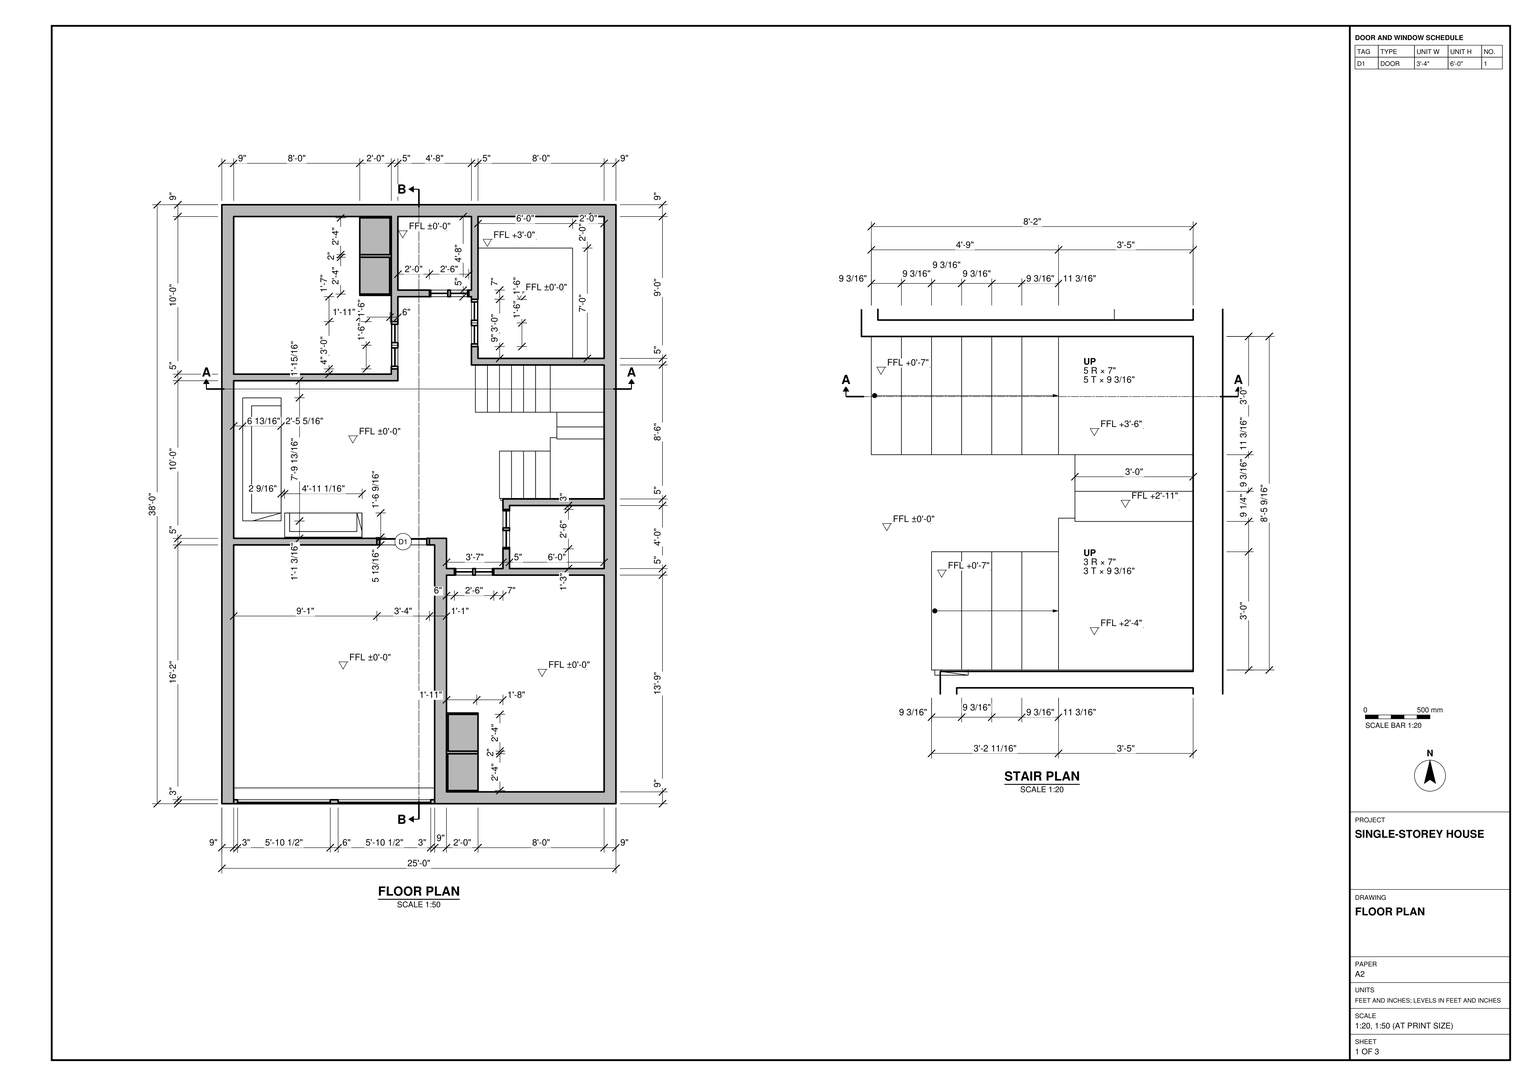
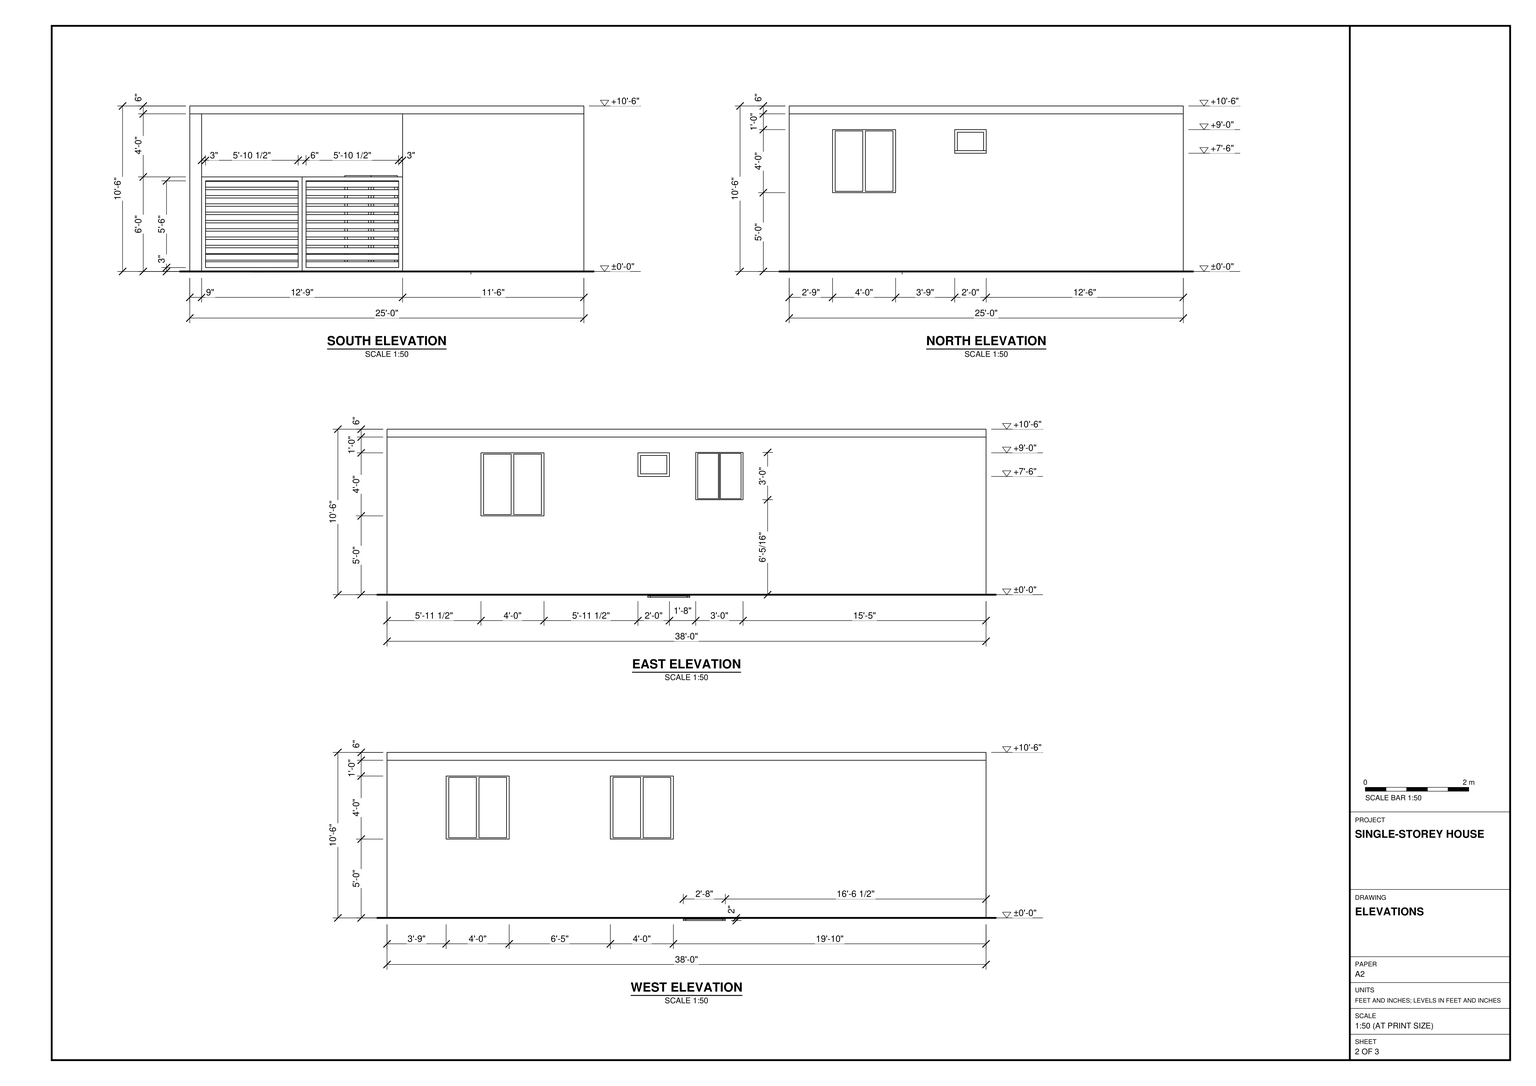
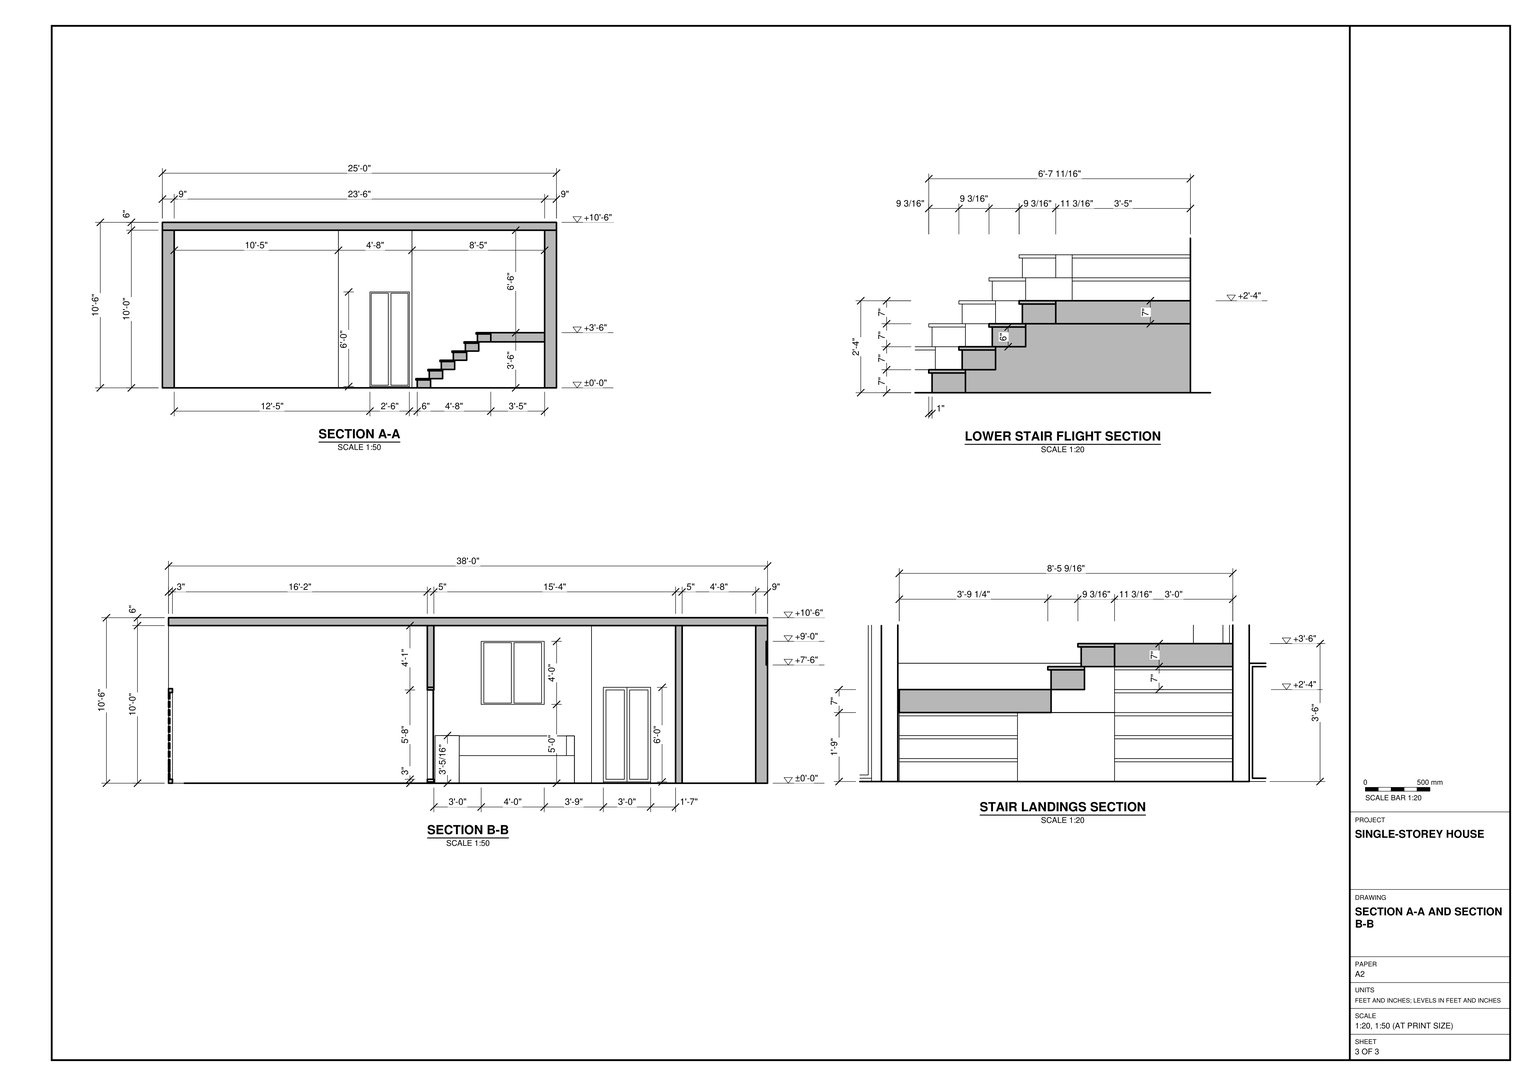
Build the single-storey house in SketchUp using task_files/diagram_01.pdf. Work in feet and inches. Set the ground-floor level at ±0'-0". The house measures 25'-0" east to west and 38'-0" north to south, with an overall model height of 10'-8".

Use the floor plan to lay out the two large southern rooms, the central space, the northern rooms and the small room immediately south of the stairs. Model the floor slab, walls at their drawn thicknesses, and flat roof slab. Fit the scheduled door in the partition between the southwest room and the central space. Use the elevations to position the windows and the paired slatted panels on the south face.

Build the two stair flights on the east side of the central space. Follow the enlarged plan and sections for the treads, risers and steps connecting the landings. Include the raised area in the northeast room, the low units arranged at right angles in the central space and the paired rectangular units in the northwest and southeast rooms.

Keep shell elements such as walls, slabs and roof, and each furniture or joinery piece, in separate groups or components. Use components for repeated parts. Decor and loose items may be represented by any suitable library component. Save one SketchUp model as output_files/single_storey_house_with_paired_stair_flights.skp.

# SketchUp Ruby script. Lengths in inches.
U = 1.inch
M = Sketchup.active_model
def pt(a) = Geom::Point3d.new(a.map { |v| v * U })
def face(e, loops, mat)
  f = e.add_face(loops[0].map { |a| pt(a) })
  loops[1..].each { |l| e.add_face(l.map { |a| pt(a) }).erase! }
  f.material = f.back_material = mat if mat
  f
end
# faces: each face lists its corners as indices into pts; further lists are holes
def faces(e, pts, list, mat = nil) = list.each { |f| face(e, (f[0].is_a?(Array) ? f : [f]).map { |l| l.map { |i| pts[i] } }, mat) }
# xy, xz, yz: faces in a plane at the given z, y or x. An outline is a flat list of corners, or four numbers for a rectangle; further outlines are holes
def ring(l) = l.size == 4 ? [[l[0], l[1]], [l[2], l[1]], [l[2], l[3]], [l[0], l[3]]] : l.each_slice(2).to_a
def flat(e, list, mat, &to3) = list.each { |f| face(e, (f[0].is_a?(Array) ? f : [f]).map { |l| ring(l).map { |u, v| to3.(u, v) } }, mat) }
def xy(e, z, list, mat = nil) = flat(e, list, mat) { |x, y| [x, y, z] }
def xz(e, y, list, mat = nil) = flat(e, list, mat) { |x, z| [x, y, z] }
def yz(e, x, list, mat = nil) = flat(e, list, mat) { |y, z| [x, y, z] }
def lines(e, pts, list) = list.each { |a, b| e.add_line(pt(pts[a]), pt(pts[b])) }
# prism: a flat outline (further loops are holes) pulled along v
def prism(e, loops, v, mat = nil)
  f = face(e, loops, mat); d = Geom::Vector3d.new(v.map { |x| x * U })
  f.pushpull(f.normal.samedirection?(d) ? d.length : -d.length)
end
def box(e, o, s, mat = nil) = prism(e, [[o, [o[0] + s[0], o[1], o[2]], [o[0] + s[0], o[1] + s[1], o[2]], [o[0], o[1] + s[1], o[2]]]], [0, 0, s[2]], mat)
def at(x, y, z, deg = 0) = Geom::Transformation.translation(pt([x, y, z])) * Geom::Transformation.rotation(ORIGIN, Z_AXIS, deg.degrees)
def axes(o, x, y, z) = Geom::Transformation.new([*x, 0, *y, 0, *z, 0, *pt(o).to_a, 1])
def part(name) = M.definitions.add(name)
# library, detail: a bought-in or finely detailed component or shape, given as its bounding box
def library(name, o, s) = part(name).tap { |d| box(d.entities, o, s) }
def detail(e, o, s) = box(e.add_group.entities, o, s)
def put(e, d, t, mat = nil) = e.add_instance(d, t).tap { |i| i.material = mat if mat }
def group(e, t, mat = nil) = e.add_group.tap { |g| g.transformation = t; g.material = mat if mat }.entities
root = M.entities
M.materials.add("[Blinds Vertical Pattern]").color = [212, 212, 214]
M.materials.add("[Blinds Vertical Stripe Gray]").color = [160, 160, 160]
M.materials.add("[Blinds Wood Light]").color = [155, 100, 14]
M.materials.add("[Field Square Tile]").color = [217, 201, 169]
M.materials.add("[Granite Tile]").color = [155, 148, 143]
M.materials.add("[Marble Carrara Floor Tile]").color = [204, 208, 219]
M.materials.add("[Marble Carrara Gold Floor Tile]").color = [225, 223, 217]
M.materials.add("[Metal Aluminum Anodized]").color = [202, 209, 219]
M.materials.add("[Metal Rusted]").color = [184, 117, 91]
M.materials.add("[Translucent Glass Tinted]").color = [8, 201, 241]
M.materials["[Translucent Glass Tinted]"].alpha = 0.48
M.materials.add("[Wood Cherry Original]").color = [152, 86, 42]
M.materials.add("[Wood Floor Parquet]").color = [145, 89, 39]
M.materials.add("[Wood OSB]").color = [240, 195, 122]
c1 = part("Window sill \#1")
box(c1.entities,[0,0,0],[40,5,1])
c2 = part("Two-panel window")
xy(c2.entities,0,[[0,-2.5,30,2.5]],"[Blinds Wood Light]")
xy(c2.entities,1,[[1,-2.5,14,0],[16,-2.5,29,0],[1,0,14,2.5],[16,0,29,2.5]],"[Blinds Wood Light]")
xy(c2.entities,71,[[1,-2.5,14,0],[16,-2.5,29,0],[1,0,14,2.5],[16,0,29,2.5]],"[Blinds Wood Light]")
xy(c2.entities,72,[[0,-2.5,30,2.5]],"[Blinds Wood Light]")
xz(c2.entities,-2.5,[[[0,0,30,72],[16,1,29,71],[1,1,14,71]]],"[Blinds Wood Light]")
xz(c2.entities,0,[[1,1,14,71],[16,1,29,71]],"[Blinds Wood Light]")
xz(c2.entities,2.5,[[[0,0,30,72],[16,1,29,71],[1,1,14,71]]],"[Blinds Wood Light]")
yz(c2.entities,0,[[-2.5,0,2.5,72]],"[Blinds Wood Light]")
yz(c2.entities,1,[[-2.5,1,0,71],[0,1,2.5,71]],"[Blinds Wood Light]")
yz(c2.entities,14,[[-2.5,1,0,71],[0,1,2.5,71]],"[Blinds Wood Light]")
yz(c2.entities,16,[[-2.5,1,0,71],[0,1,2.5,71]],"[Blinds Wood Light]")
yz(c2.entities,29,[[-2.5,1,0,71],[0,1,2.5,71]],"[Blinds Wood Light]")
yz(c2.entities,30,[[-2.5,0,2.5,72]],"[Blinds Wood Light]")
c3 = part("Window sill")
xy(c3.entities,0,[[0,0,30,5]],"[Marble Carrara Gold Floor Tile]")
xy(c3.entities,1,[[0,0,30,5]],"[Wood OSB]")
xz(c3.entities,0,[[0,0,30,1]],"[Wood OSB]")
xz(c3.entities,5,[[0,0,30,1]],"[Wood OSB]")
yz(c3.entities,0,[[0,0,5,1]],"[Marble Carrara Gold Floor Tile]")
yz(c3.entities,30,[[0,0,5,1]],"[Marble Carrara Gold Floor Tile]")
c4 = part("Window sash")
xy(c4.entities,0,[[0,0,1,24]],"[Blinds Vertical Pattern]")
xy(c4.entities,2,[[0,2,1,22]],"[Blinds Vertical Pattern]")
xy(c4.entities,16,[[0,2,1,22]],"[Blinds Vertical Pattern]")
xy(c4.entities,18,[[0,0,1,24]],"[Blinds Vertical Pattern]")
xz(c4.entities,0,[[0,0,1,18]],"[Blinds Vertical Pattern]")
xz(c4.entities,2,[[0,2,1,16]],"[Blinds Vertical Pattern]")
xz(c4.entities,22,[[0,2,1,16]],"[Blinds Vertical Pattern]")
xz(c4.entities,24,[[0,0,1,18]],"[Blinds Vertical Pattern]")
yz(c4.entities,0,[[[0,0,24,18],[2,2,22,16]]],"[Blinds Vertical Pattern]")
yz(c4.entities,0,[[2,2,22,16]],"[Blinds Vertical Stripe Gray]")
yz(c4.entities,1,[[[0,0,24,18],[2,2,22,16]]],"[Blinds Vertical Pattern]")
c5 = part("Stair step")
xy(c5.entities,0,[[0,0,10.17,36]],"[Marble Carrara Gold Floor Tile]")
xy(c5.entities,6,[[0,0,10.17,36]],"[Granite Tile]")
xz(c5.entities,0,[[0,0,10.17,6]],"[Granite Tile]")
xz(c5.entities,36,[[0,0,10.17,6]],"[Marble Carrara Gold Floor Tile]")
yz(c5.entities,0,[[0,0,36,6]],"[Granite Tile]")
yz(c5.entities,10.17,[[0,0,36,6]],"[Granite Tile]")
c6 = part("Group\#4")
xy(c6.entities,0,[[0,-3.5,48,5.5]])
xy(c6.entities,1,[[2,-3.5,23,1],[25,-3.5,46,1],[2,1,23,5.5],[25,1,46,5.5]],"[Wood Cherry Original]")
xy(c6.entities,47,[[2,-3.5,23,1],[25,-3.5,46,1],[2,1,23,5.5],[25,1,46,5.5]],"[Wood Cherry Original]")
xy(c6.entities,48,[[0,-3.5,48,5.5]],"[Wood Cherry Original]")
xz(c6.entities,-3.5,[[[0,0,48,48],[2,1,23,47],[25,1,46,47]]],"[Wood Cherry Original]")
xz(c6.entities,1,[[2,1,23,47],[25,1,46,47]],"[Translucent Glass Tinted]")
xz(c6.entities,5.5,[[[0,0,48,48],[2,1,23,47],[25,1,46,47]]],"[Wood Cherry Original]")
yz(c6.entities,0,[[-3.5,0,5.5,48]],"[Wood Cherry Original]")
yz(c6.entities,2,[[-3.5,1,1,47],[1,1,5.5,47]],"[Wood Cherry Original]")
yz(c6.entities,23,[[-3.5,1,1,47],[1,1,5.5,47]],"[Wood Cherry Original]")
yz(c6.entities,25,[[-3.5,1,1,47],[1,1,5.5,47]],"[Wood Cherry Original]")
yz(c6.entities,46,[[-3.5,1,1,47],[1,1,5.5,47]],"[Wood Cherry Original]")
yz(c6.entities,48,[[-3.5,0,5.5,48]],"[Wood Cherry Original]")
c7 = part("Framing strip")
box(c7.entities,[0,-1,-2],[70.5,1,4.41])
c8 = part("Group\#1")
g1 = group(c8.entities,at(0,0,0))
xy(g1,0,[[0,0,5,36]],"[Marble Carrara Gold Floor Tile]")
xy(g1,1,[[0,0,5,36]],"[Wood OSB]")
xz(g1,0,[[0,0,5,1]],"[Marble Carrara Gold Floor Tile]")
xz(g1,36,[[0,0,5,1]],"[Marble Carrara Gold Floor Tile]")
yz(g1,0,[[0,0,36,1]],"[Wood OSB]")
yz(g1,5,[[0,0,36,1]],"[Wood OSB]")
c9 = part("Group\#9")
box(c9.entities,[-1,0,0],[11.17,36,1])
c10 = part("Rectangular panel")
box(c10.entities,[1,-28,0],[22,28,1])
c11 = part("Group\#14")
yz(c11.entities,0,[[0,0,28,70]])
c12 = part("Group\#13")
xy(c12.entities,0,[[-24,0,0,60]])
xy(c12.entities,1,[[-24,1,-1.25,29],[-24,31,-1,59]])
xy(c12.entities,71,[[-24,1,-1.25,29],[-24,31,-1,59]])
xy(c12.entities,72,[[-24,0,0,60]])
xz(c12.entities,0,[[-24,0,0,72]])
xz(c12.entities,1,[[-24,1,-1.25,71]])
xz(c12.entities,29,[[-24,1,-1.25,71]])
xz(c12.entities,31,[[-24,1,-1,71]])
xz(c12.entities,59,[[-24,1,-1,54.74],[-24,54.74,-1,55.74],[-24,55.74,-1,71]])
xz(c12.entities,60,[[-24,0,0,72]])
yz(c12.entities,-24,[[[0,0,60,72],[1,1,29,71],[31,1,59,71]]])
yz(c12.entities,-1.25,[[1,1,29,71]])
yz(c12.entities,-1,[[31,1,59,71]])
yz(c12.entities,0,[[0,0,60,72]])
p = [[-24,29.99,-0.01],[-24,29.99,0],[-24,60.01,72.01],[-24,60.01,-0.01],[-24,29.99,72],[-24,29.99,72.01]]
lines(c12.entities,p,[[0,1],[2,3],[3,0],[4,5]])
put(c12.entities,c10,at(-24,59,70))
put(c12.entities,c10,at(-24,59,56.2))
put(c12.entities,c10,at(-24,59,42.4))
put(c12.entities,c10,at(-24,59,28.6))
put(c12.entities,c10,at(-24,59,14.8))
put(c12.entities,c10,at(-24,59,1))
put(c12.entities,c10,at(-24,29,56.2))
put(c12.entities,c10,at(-24,29,42.4))
put(c12.entities,c10,at(-24,29,14.8))
put(c12.entities,c10,at(-24,29,28.6))
put(c12.entities,c10,at(-24,29,1))
put(c12.entities,c10,at(-24,29,70))
put(c12.entities,c11,at(-24,31,1))
put(c12.entities,c11,at(-24,1,1))
xy(root,0,[[0,0,9,0,9,197,162,197,162,0,300,0,300,191,291,191,291,179,219,179,219,194,214,194,214,179,207,179,207,174,291,174,291,9,171,9,171,174,177,174,177,179,171,179,171,202,9,202,9,238,0,238],[0,286,9,286,9,322,134,322,134,331,129,331,129,327,9,327,9,447,129,447,129,367,134,367,134,386,158,386,158,391,134,391,134,447,150,447,150,456,0,456]])
xy(root,0,[[219,179,291,227]],"[Marble Carrara Floor Tile]")
xy(root,0,[[171,9,291,9,291,174,207,174,207,179,214,179,214,232,222.5,230.84,212.33,230.84,212.33,266.84,214.33,266.84,214.33,268,222.5,266.84,222.5,232,291,232,291,334,204.17,334,204.17,298,194,298,194,334,190,334,190,348,195,348,195,339,267,339,267,423,195,423,195,384,190,384,190,386,134,386,134,322,9,322,9,202,171,202,171,179,177,179,177,174,171,174],[9,12,162,197],[291,215,300,215,300,456,291,456,291,339,195,339,195,348,190,348,190,334,244.83,334,244.83,334.07,255.375,334.07,255.375,334,291,334,291,232,222.5,232,222.5,230.84,214,232,214,224,219,224,219,227,291,227],[212.33,230.84,222.5,230.84,214,232,214.33,232,214.33,266.84,212.33,266.84],[222.5,230.84,222.5,232,214,232],
  [214.33,232,222.5,266.84],[214.33,266.84,214.33,268,222.5,266.84],[194,298,204.17,334],[9,327,129,447],[244.83,334,255.375,334.07],
  [190,384,195,384,195,456,174,456,174,447,190,447,190,391,188,391,188,386,190,386],[134,391,190,447]],"[Marble Carrara Gold Floor Tile]")
xy(root,1,[[267,340,290,360],[267,361,290,380.5],[267,381.5,290,401],[267,402,290,422],[196,423,218.83,446],
  [219.83,423,242.17,446],[243.17,423,266,446]],"[Field Square Tile]")
xy(root,35,[[267,340,290,360],[267,361,290,380.5],[267,381.5,290,401],[267,402,290,422],[196,423,218.83,446],
  [219.83,423,242.17,446],[243.17,423,266,446]],"[Field Square Tile]")
xy(root,36,[[267,339,291,339,291,447,195,447,195,423,267,423]],"[Field Square Tile]")
xy(root,60,[[291,71.5,300,119.5],[0,238,9,286],[0,363,9,411],[219,447,267,456]])
xy(root,72.31,[[291,235,300,271]])
xy(root,73,[[177,174,207,179],[214,194,219,224],[118,197,158,202],[129,331,134,367],[190,348,195,384],
  [158,386,188,391]])
xy(root,90,[[291,191,300,215]])
xy(root,92,[[150,447,174,456]])
xy(root,108,[[291,71.5,300,119.5],[291,191,300,215],[0,238,9,286],[0,363,9,411],[150,447,174,456],
  [219,447,267,456]])
xy(root,108.31,[[291,235,300,271]])
xy(root,120,[[[0,0,9,0,9,197,162,197,162,0,300,0,300,456,0,456],[171,179,171,202,9,202,9,322,134,322,134,386,190,386,190,334,291,334,291,232,214,232,214,179],[171,9,291,174],[9,327,129,447],[195,339,291,447],[219,179,291,227],[134,391,190,447]]])
xz(root,0,[[0,0,9,120],[162,0,300,120]])
xz(root,9,[[171,0,291,120]])
xz(root,71.5,[[291,60,300,108]])
xz(root,119.5,[[291,60,300,108]])
xz(root,174,[[171,0,177,0,177,73,207,73,207,0,291,0,291,120,171,120]])
xz(root,179,[[171,0,171,120,214,120,214,0,207,0,207,73,177,73,177,0],[219,0,291,120]])
xz(root,191,[[291,90,300,108]])
xz(root,194,[[214,0,219,73]])
xz(root,197,[[9,0,118,0,118,73,158,73,158,0,162,0,162,120,9,120]])
xz(root,202,[[9,0,9,120,171,120,171,0,158,0,158,73,118,73,118,0]])
xz(root,215,[[291,90,300,108]])
xz(root,224,[[214,0,219,73]])
xz(root,227,[[219,0,291,120]])
xz(root,232,[[214,0,291,120]])
xz(root,235,[[291,72.31,300,108.31]])
xz(root,238,[[0,60,9,108]])
xz(root,271,[[291,72.31,300,108.31]])
xz(root,286,[[0,60,9,108]])
xz(root,322,[[9,0,134,120]])
xz(root,327,[[9,0,129,120]])
xz(root,331,[[129,0,134,73]])
xz(root,334,[[190,0,291,120]])
xz(root,339,[[195,0,195,120,291,120,291,36,267,36,267,0]])
xz(root,339,[[267,0,291,36]],"[Marble Carrara Gold Floor Tile]")
xz(root,340,[[267,1,290,35]],"[Field Square Tile]")
xz(root,348,[[190,0,195,73]])
xz(root,360,[[267,1,290,35]],"[Field Square Tile]")
xz(root,361,[[267,1,290,35]],"[Field Square Tile]")
xz(root,363,[[0,60,9,108]])
xz(root,367,[[129,0,134,73]])
xz(root,380.5,[[267,1,290,35]],"[Field Square Tile]")
xz(root,381.5,[[267,1,290,35]],"[Field Square Tile]")
xz(root,384,[[190,0,195,73]])
xz(root,386,[[134,0,158,0,158,73,188,73,188,0,190,0,190,120,134,120]])
xz(root,391,[[134,0,134,120,188,120,188,73,158,73,158,0],[188,0,190,120]])
xz(root,401,[[267,1,290,35]],"[Field Square Tile]")
xz(root,402,[[267,1,290,35]],"[Field Square Tile]")
xz(root,411,[[0,60,9,108]])
xz(root,422,[[267,1,290,35]],"[Field Square Tile]")
xz(root,423,[[[195,0,267,36],[196,1,218.83,35],[243.17,1,266,35],[219.83,1,242.17,35]]],"[Field Square Tile]")
xz(root,446,[[196,1,218.83,35],[219.83,1,242.17,35],[243.17,1,266,35]],"[Field Square Tile]")
xz(root,447,[[9,0,129,120],[[134,0,190,120],[150,92,174,108]],[195,36,219,36,219,108,267,108,267,36,291,36,291,120,195,120]])
xz(root,447,[[219,36,267,60]],"[Marble Carrara Gold Floor Tile]")
xz(root,456,[[[0,0,300,120],[219,60,267,108],[150,92,174,108]]])
yz(root,0,[[[0,0,456,120],[363,60,411,108],[238,60,286,108]]])
yz(root,9,[[0,0,197,120],[[202,0,322,120],[238,60,286,108]],[[327,0,447,120],[363,60,411,108]]])
yz(root,118,[[197,-0.25,202,72],[197,72,202,73]])
yz(root,129,[[327,0,327,120,447,120,447,72,387,72,387,0,367,0,367,73,331,73,331,0]])
yz(root,134,[[322,0,331,0,331,73,367,73,367,0,386,0,386,120,322,120],[391,0,447,120]])
yz(root,150,[[447,92,456,108]])
yz(root,158,[[197,-0.25,202,72],[386,0,391,73],[197,72,202,73]])
yz(root,162,[[0,0,197,120]])
yz(root,171,[[9,0,174,120],[179,0,202,120]])
yz(root,174,[[447,92,456,108]])
yz(root,177,[[174,0,179,73]])
yz(root,188,[[386,0,391,73]])
yz(root,190,[[334,0,334,120,386,120,386,0,384,0,384,73,348,73,348,0],[391,0,447,120]])
yz(root,195,[[339,0,348,120],[384,0,423,0,423,36,447,36,447,120,348,120,348,73,384,73]])
yz(root,195,[[423,0,447,36]],"[Marble Carrara Gold Floor Tile]")
yz(root,196,[[423,1,446,35]],"[Field Square Tile]")
yz(root,207,[[174,0,179,73]])
yz(root,214,[[198.48,-2,200.48,-1],[200.48,-2,228.48,-1],[228.48,-2,230.48,-1],[179,0,179,120,232,120,232,0,224,0,224,73,194,73,194,0]])
yz(root,218.83,[[423,1,446,35]],"[Field Square Tile]")
yz(root,219,[[179,0,194,0,194,73,224,73,224,0,227,0,227,120,179,120],[447,60,456,108]])
yz(root,219.83,[[423,1,446,35]],"[Field Square Tile]")
yz(root,242.17,[[423,1,446,35]],"[Field Square Tile]")
yz(root,243.17,[[423,1,446,35]],"[Field Square Tile]")
yz(root,266,[[423,1,446,35]],"[Field Square Tile]")
yz(root,267,[[447,60,456,108]])
yz(root,267,[[[339,0,423,36],[340,1,422,35]],[360,1,361,35],[380.5,1,381.5,35],[401,1,402,35]],"[Field Square Tile]")
yz(root,290,[[340,1,360,35],[361,1,380.5,35],[381.5,1,401,35],[402,1,422,35]],"[Field Square Tile]")
yz(root,291,[[[9,0,174,120],[71.5,60,119.5,108]],[[179,0,227,120],[191,90,215,108]],[[232,0,334,120],[235,72.31,271,108.31]],[339,36,447,120]])
yz(root,291,[[339,0,447,36]],"[Marble Carrara Gold Floor Tile]")
yz(root,300,[[[0,0,456,120],[71.5,60,119.5,108],[235,72.31,271,108.31],[191,90,215,108]]])
p = [[300,253,108.31],[300,253,72.31],[118,202,72],[158,202,72],[129.5,351,3],[129.5,347,3],
  [129,364.89,1],[129.5,365,3],[204.17,298,7],[203.17,298,7]]
lines(root,p,[[0,1],[2,3],[4,5],[6,7],[8,9]])
put(root,c1,at(118,197,0),"[Wood OSB]")
put(root,c2,at(216.5,224,1,-90))
put(root,c2,at(158,388.5,1))
put(root,c3,at(158,386,0))
put(root,c3,at(219,194,0,90))
put(root,c4,at(299,191,90))
put(root,c4,at(174,455,90,90))
put(root,c2,at(207,176.5,1,-180))
put(root,c3,at(177,174,0))
put(root,c5,at(194,298,0),"[Granite Tile]")
put(root,c5,at(203.17,298,7),"[Granite Tile]")
put(root,c5,at(212.33,298,14),"[Granite Tile]")
put(root,c5,at(221.5,298,21),"[Granite Tile]")
put(root,c5,at(230.67,298,28),"[Granite Tile]")
put(root,c5,at(239.83,298,35),"[Granite Tile]")
put(root,c5,at(291,287.83,35,90),"[Granite Tile]")
put(root,c5,at(291,278.67,28,90),"[Granite Tile]")
put(root,c5,at(239.83,232.4375,21),"[Granite Tile]")
put(root,c5,at(221.5,232.4375,7),"[Granite Tile]")
put(root,c5,at(230.67,232.4375,14),"[Granite Tile]")
put(root,c5,at(212.33,232.4375,0),"[Granite Tile]")
put(root,c6,at(3.5,286,60,-90))
put(root,c6,at(3.5,411,60,-90))
put(root,c6,at(219,450.5,60))
put(root,c6,at(294.5,119.5,60,-90))
g2 = group(root,at(9,-9,0))
xy(g2,0,[[0,9,153,12]])
xy(g2,3,[[3,9,73.5,12],[79.5,9,150,12]],"[Metal Aluminum Anodized]")
xy(g2,69,[[79.5,9,150,12]])
xy(g2,69,[[3,9,73.5,12]],"[Metal Aluminum Anodized]")
xy(g2,72,[[0,9,76.5,12],[76.5,9,153,12]],"[Metal Aluminum Anodized]")
xz(g2,9,[[[0,0,76.5,72],[3,3,73.5,69]],[[76.5,0,153,72],[79.5,3,150,69]]],"[Metal Aluminum Anodized]")
xz(g2,12,[[[0,0,153,72],[3,3,73.5,69],[79.5,3,150,69]]],"[Metal Aluminum Anodized]")
yz(g2,0,[[9,0,12,72]])
yz(g2,3,[[9,3,12,69]],"[Metal Aluminum Anodized]")
yz(g2,73.5,[[9,3,12,69]],"[Metal Aluminum Anodized]")
yz(g2,79.5,[[9,3,12,69]])
yz(g2,150,[[9,3,12,69]],"[Metal Aluminum Anodized]")
yz(g2,153,[[9,0,12,72]])
put(g2,c7,at(3,10,66.15),"[Metal Rusted]")
put(g2,c7,at(3,10,59.83),"[Metal Rusted]")
put(g2,c7,at(3,10,53.52),"[Metal Rusted]")
put(g2,c7,at(3,10,47.2),"[Metal Rusted]")
put(g2,c7,at(3,10,40.89),"[Metal Rusted]")
put(g2,c7,at(3,10,34.57),"[Metal Rusted]")
put(g2,c7,at(3,10,28.26),"[Metal Rusted]")
put(g2,c7,at(3,10,21.94),"[Metal Rusted]")
put(g2,c7,at(3,10,15.63),"[Metal Rusted]")
put(g2,c7,at(3,10,10.62),"[Metal Rusted]")
put(g2,c7,at(3,10,5),"[Metal Rusted]")
put(g2,c7,at(79.5,10,40.89),"[Metal Rusted]")
put(g2,c7,at(79.5,10,10.62),"[Metal Rusted]")
put(g2,c7,at(79.5,10,28.26),"[Metal Rusted]")
put(g2,c7,at(79.5,10,15.63),"[Metal Rusted]")
put(g2,c7,at(79.5,10,53.52),"[Metal Rusted]")
put(g2,c7,at(79.5,10,59.83),"[Metal Rusted]")
put(g2,c7,at(79.5,10,5),"[Metal Rusted]")
put(g2,c7,at(79.5,10,66.15),"[Metal Rusted]")
put(g2,c7,at(79.5,10,47.2),"[Metal Rusted]")
put(g2,c7,at(79.5,10,34.57),"[Metal Rusted]")
put(g2,c7,at(79.5,10,21.94),"[Metal Rusted]")
g3 = group(root,at(293.25,235,72.31))
xy(g3,0,[[0,0,6.75,36]])
xy(g3,0.75,[[0,1.5,3.375,17.25],[3.375,1.5,6.75,17.25],[0,18.75,3.375,34.5],[3.375,18.75,6.75,34.5]],"[Wood Cherry Original]")
xy(g3,35.25,[[0,1.5,3.375,17.25],[3.375,1.5,6.75,17.25],[0,18.75,3.375,34.5],[3.375,18.75,6.75,34.5]],"[Wood Cherry Original]")
xy(g3,36,[[0,0,6.75,36]],"[Wood Cherry Original]")
xz(g3,0,[[0,0,6.75,36]],"[Wood Cherry Original]")
xz(g3,1.5,[[0,0.75,3.375,35.25],[3.375,0.75,6.75,35.25]],"[Wood Cherry Original]")
xz(g3,17.25,[[0,0.75,3.375,35.25],[3.375,0.75,6.75,35.25]],"[Wood Cherry Original]")
xz(g3,18.75,[[0,0.75,3.375,35.25],[3.375,0.75,6.75,35.25]],"[Wood Cherry Original]")
xz(g3,34.5,[[0,0.75,3.375,35.25],[3.375,0.75,6.75,35.25]],"[Wood Cherry Original]")
xz(g3,36,[[0,0,6.75,36]],"[Wood Cherry Original]")
yz(g3,0,[[[0,0,36,36],[18.75,0.75,34.5,35.25],[1.5,0.75,17.25,35.25]]],"[Wood Cherry Original]")
yz(g3,3.375,[[1.5,0.75,17.25,35.25],[18.75,0.75,34.5,35.25]],"[Translucent Glass Tinted]")
yz(g3,6.75,[[[0,0,36,36],[18.75,0.75,34.5,35.25],[1.5,0.75,17.25,35.25]]],"[Wood Cherry Original]")
g4 = group(root,at(118,197,1))
xy(g4,2,[[2,0,18,4.5],[22,0,38,4.5],[2,4.5,18,5],[22,4.5,38,5]],"[Wood Floor Parquet]")
xy(g4,70,[[2,0,18,4.5],[22,0,38,4.5],[2,4.5,18,5],[22,4.5,38,5]])
xy(g4,72,[[0,0,20,5],[20,0,40,5]],"[Wood Floor Parquet]")
xz(g4,0,[[[0,0,20,72],[2,2,18,70]],[[20,0,40,72],[22,2,38,70]]],"[Wood Floor Parquet]")
xz(g4,4.5,[[2,2,18,70],[22,2,38,70]],"[Wood Floor Parquet]")
xz(g4,5,[[0,0,2,70],[2,0.05,38,2],[38,0.05,40,72],[18,2,22,72],[0,70,18,72],
  [22,70,38,72]],"[Wood Floor Parquet]")
yz(g4,0,[[0,0,5,72]],"[Wood Floor Parquet]")
yz(g4,2,[[0,2,4.5,70],[4.5,2,5,70]],"[Wood Floor Parquet]")
yz(g4,18,[[4.5,2,5,70]])
yz(g4,18,[[0,2,4.5,70]],"[Wood Floor Parquet]")
yz(g4,22,[[0,2,4.5,70],[4.5,2,5,70]],"[Wood Floor Parquet]")
yz(g4,38,[[4.5,2,5,70]])
yz(g4,38,[[0,2,4.5,70]],"[Wood Floor Parquet]")
yz(g4,40,[[0,0.05,5,72]],"[Wood Floor Parquet]")
g5 = group(root,at(127.6875,400.375,1),"[Wood Floor Parquet]")
xy(g5,0,[[1.8125,-69.375,6.3125,-53.77],[1.8125,-53.77,6.3125,-51.375],[1.8125,-51.375,6.3125,-33.375]])
xy(g5,2,[[1.8125,-67.375,4.0625,-53.375],[4.0625,-67.375,6.3125,-53.375],[1.8125,-49.375,4.0625,-35.375],[4.0625,-49.375,6.3125,-35.375]])
xy(g5,70,[[1.8125,-67.375,4.0625,-53.375],[4.0625,-67.375,6.3125,-53.375],[1.8125,-49.375,4.0625,-35.375],[4.0625,-49.375,6.3125,-35.375]])
xy(g5,72,[[1.8125,-69.375,6.3125,-51.375],[1.8125,-51.375,6.3125,-33.375]])
xz(g5,-69.375,[[1.8125,0,6.3125,72]])
xz(g5,-67.375,[[1.8125,2,4.0625,70],[4.0625,2,6.3125,70]])
xz(g5,-53.375,[[1.8125,2,4.0625,70],[4.0625,2,6.3125,70]])
xz(g5,-49.375,[[1.8125,2,4.0625,70],[4.0625,2,6.3125,70]])
xz(g5,-35.375,[[1.8125,2,4.0625,70],[4.0625,2,6.3125,70]])
xz(g5,-33.375,[[1.8125,0,6.3125,72]])
yz(g5,1.3125,[[-69.375,0,-67.22,72],[-35.48,0,-33.375,72],[-49.375,70,-49.375,72,-48.86,72,-48.86,70.68,-35.48,70.68,-35.48,70],[-48.86,70.68,-35.48,72]])
yz(g5,4.0625,[[-67.375,2,-53.375,70],[-49.375,2,-35.375,70]])
yz(g5,6.3125,[[[-69.375,0,-51.375,72],[-67.375,2,-53.375,70]],[[-51.375,0,-33.375,72],[-49.375,2,-35.375,70]]])
p = [[1.8125,-53.375,70],[1.3125,-67.22,70],[1.3125,-67.22,72],[1.8125,-53.375,72],[1.3125,-35.48,70],[1.8125,-49.375,70],
  [1.8125,-49.375,72],[1.3125,-35.48,72],[1.3125,-35.48,70.68]]
faces(g5,p,[[0,1,2,3],[4,5,6,7,8]])
g6 = group(root,at(196.3125,314.625,1,180),"[Wood Floor Parquet]")
xy(g6,0,[[1.8125,-69.375,6.3125,-51.375],[1.8125,-51.375,6.3125,-33.375]])
xy(g6,2,[[1.8125,-67.375,4.0625,-53.375],[4.0625,-67.375,6.3125,-53.375],[1.8125,-49.375,4.0625,-35.375],[4.0625,-49.375,6.3125,-35.375]])
xy(g6,70,[[1.8125,-67.375,4.0625,-53.375],[4.0625,-67.375,6.3125,-53.375],[1.8125,-49.375,4.0625,-35.375],[4.0625,-49.375,6.3125,-35.375]])
xy(g6,72,[[1.8125,-69.375,6.3125,-51.375],[1.8125,-51.375,6.3125,-33.375]])
xz(g6,-69.375,[[1.8125,0,6.3125,72]])
xz(g6,-67.375,[[1.8125,2,4.0625,70],[4.0625,2,6.3125,70]])
xz(g6,-53.375,[[1.8125,2,4.0625,70],[4.0625,2,6.3125,70]])
xz(g6,-49.375,[[1.8125,2,4.0625,70],[4.0625,2,6.3125,70]])
xz(g6,-35.375,[[1.8125,2,4.0625,70],[4.0625,2,6.3125,70]])
xz(g6,-33.375,[[1.8125,0,6.3125,72]])
yz(g6,4.0625,[[-67.375,2,-53.375,70],[-49.375,2,-35.375,70]])
yz(g6,6.3125,[[[-69.375,0,-51.375,72],[-67.375,2,-53.375,70]],[[-51.375,0,-33.375,72],[-49.375,2,-35.375,70]]])
put(root,c8,at(129,331,0),"[Wood OSB]")
put(root,c8,at(195,384,0,180),"[Wood OSB]")
put(root,c9,at(194,298,6),"[Granite Tile]")
put(root,c9,at(203.17,298,13),"[Granite Tile]")
put(root,c9,at(212.33,298,20),"[Granite Tile]")
put(root,c9,at(221.5,298,27),"[Granite Tile]")
put(root,c9,at(230.67,298,34),"[Granite Tile]")
put(root,c9,at(239.83,298,41),"[Granite Tile]")
g7 = group(root,at(250,232,35),"[Granite Tile]")
box(g7,[0,66,0],[41,36,7])
put(root,c9,at(291,287.83,41,90),"[Granite Tile]")
put(root,c9,at(291,278.67,34,90),"[Granite Tile]")
g8 = group(root,at(250,166.4375,21),"[Granite Tile]")
box(g8,[0,66,0],[41,46.23,7])
put(root,c9,at(212.33,232.4375,6),"[Granite Tile]")
put(root,c9,at(239.83,232.4375,27),"[Granite Tile]")
put(root,c9,at(230.67,232.4375,20),"[Granite Tile]")
put(root,c9,at(221.5,232.4375,13),"[Granite Tile]")
g9 = group(root,at(0,0,120))
box(g9,[0,0,0],[300,456,6])
put(root,c12,at(129,387,0))
put(root,c12,at(171,69,0,180))
g10 = group(root,at(15.84,215.3125,0))
xy(g10,0,[[0,0,0,93.625,29.25,93.625,29.25,6.01,7.69,0],[7.69,0,29.25,6.01,29.25,0]],"[Marble Carrara Gold Floor Tile]")
xy(g10,21.04,[[29.3,6.01,29.3,87.62,29.25,87.62],[29.25,87.62,29.25,93.625,29.3,87.62]])
xy(g10,36,[[7.69,0,29.25,6.01,29.25,0]])
xz(g10,0,[[0,0,29.25,36]],"[Marble Carrara Gold Floor Tile]")
xz(g10,6.01,[[6.8125,20.96,6.76,36.02,29.25,36.1,29.25,21.04],[29.25,21.04,29.25,36,29.3,21.04]])
xz(g10,87.62,[[6.8125,20.96,29.25,21.04,29.3,21.04,29.25,36,29.25,36.1,6.76,36.02]])
xz(g10,93.625,[[0,36,6.76,36.02,29.25,36.1,29.25,36]])
xz(g10,93.625,[[0,0,29.25,36]],"[Marble Carrara Gold Floor Tile]")
yz(g10,0,[[0,0,93.625,36]],"[Marble Carrara Gold Floor Tile]")
yz(g10,29.25,[[0,0,6.01,36],[87.62,36,93.625,36.1]])
yz(g10,29.25,[[-0.1,-0.1,93.73,-0.1,93.73,36.1,93.625,36.1,93.625,0,0,0,0,36,6.01,36,6.01,36.1,-0.1,36.1]],"[Marble Carrara Gold Floor Tile]")
p = [[29.3,6.01,21.04],[29.3,6.01,0],[29.25,93.625,0],[29.25,93.625,21.04],[29.25,87.62,21.04],[29.25,6.01,21.04],
  [6.8125,87.62,20.96],[6.8125,6.01,20.96],[6.76,87.62,36.02],[6.76,6.01,36.02],[29.3,87.62,21.04],[29.25,93.625,36],
  [29.25,93.625,36.1],[29.3,87.62,36.1],[0,93.625,36],[0,0,36],[29.25,0,36.1],[29.25,6.01,36.1],
  [29.25,87.62,36.1],[6.76,93.625,36.02],[6.76,93.76,36.02]]
faces(g10,p,[[0,1,2,3,4],[5,0,4,6,7],[8,9,7,6],[10,3,11,12,13],[14,15,16,17,9,8,18,12,19]])
lines(g10,p,[[19,20]])
g11 = group(root,at(106.73,202.83,0))
xz(g11,18.51,[[-58.95,36.02,-58.95,36.125,-55.18,36.14,-55.18,36.03]])
yz(g11,-58.95,[[18.51,36.02,0.13,36.09,4.375,36.09,18.51,36.125]])
p = [[-59.02,18.51,36.125],[-58.95,18.51,36.125],[-58.95,18.51,36.02],[-58.9,18.45,20.9375],[-58.82,18.38,-0.27],[-3.78,18.38,-0.08],
  [0,18.38,-0.07],[-0.13,18.51,36.23],[-3.9,18.51,36.22],[-3.9,18.51,36.32],[-0.13,18.51,36.33],[-0.0625,18.51,36.33],
  [0.07,18.38,-0.17],[-58.89,18.375,-0.38],[-58.82,0,-0.21],[-58.95,0.13,36.09],[0,4.83,-0.02],[0,0,0],
  [-3.85,18.49,21.13],[-3.78,18.41,-0.08],[-55.125,18.45,20.95],[-0.13,0.13,36.29],[-0.13,4.96,36.28],[-3.85,18.45,21.13],
  [-55.18,4.375,36.11],[-3.9,4.375,36.29],[-3.85,4.36,21.1],[-55.125,4.35,20.92],[-55.18,18.51,36.03],[-55.18,18.51,36.14],
  [-55.125,18.49,20.95],[-55.18,18.54,36.14],[-58.95,4.375,36.09],[-59.04,4.375,36.09]]
faces(g11,p,[[0,1,2,3,4,5,6,7,8,9,10,11,12,13],[4,14,15,2,3],[4,5,16,17,14],[14,17,21,15],[17,16,6,7,22,21],[6,16,5]],"[Marble Carrara Gold Floor Tile]")
faces(g11,p,[[18,19,4,3,20],[23,8,7,6,5],[24,25,26,27],[28,29,24,27,20,30],[23,18,20,27,26],[30,3,2,1,31],[3,30,20],[30,20,18],
  [9,8,23,26,25],[18,23,8],[15,21,10,9,25,24,29,1,32],[22,8,7]])
lines(g11,p,[[32,33]])
